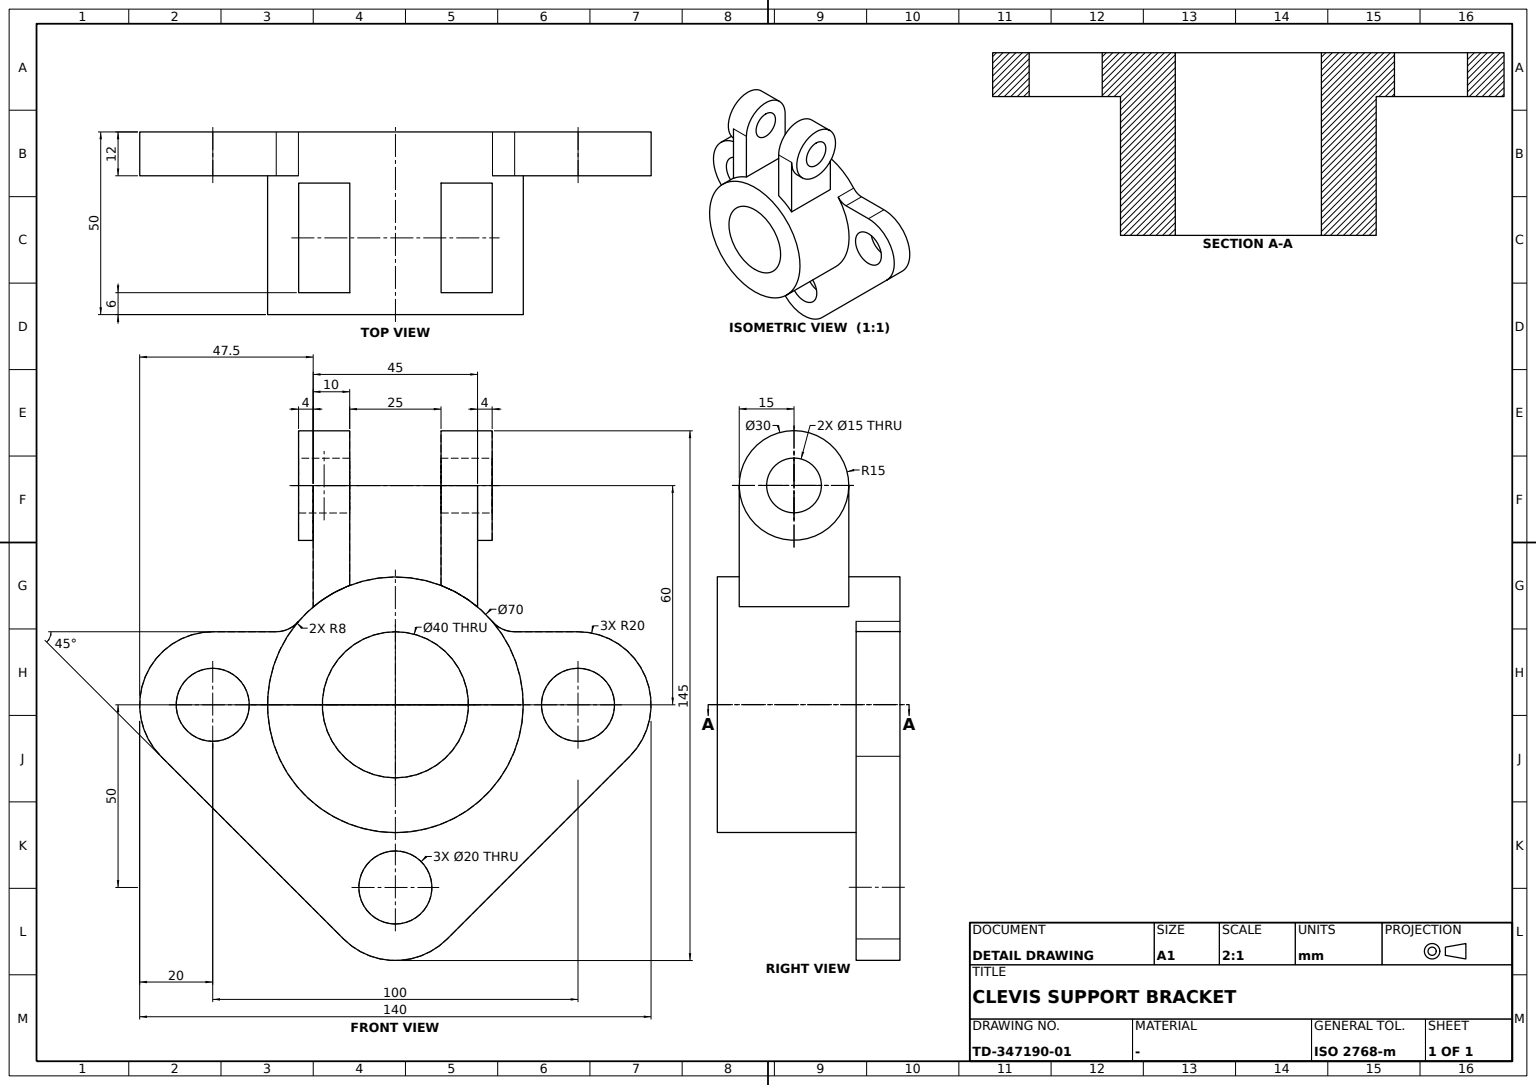
ISO-10303-21;
HEADER;
FILE_DESCRIPTION((''),'2;1');
FILE_NAME('','',(''),(''),'','','');
FILE_SCHEMA(('AUTOMOTIVE_DESIGN'));
ENDSEC;
DATA;
#1=APPLICATION_CONTEXT('');
#2=PRODUCT_CONTEXT('',#1,'mechanical');
#3=PRODUCT('','','',(#2));
#4=PRODUCT_DEFINITION_FORMATION('','',#3);
#5=PRODUCT_DEFINITION_CONTEXT('',#1,'design');
#6=PRODUCT_DEFINITION('','',#4,#5);
#7=PRODUCT_DEFINITION_SHAPE('','',#6);
#8=(LENGTH_UNIT()NAMED_UNIT(*)SI_UNIT(.MILLI.,.METRE.));
#9=(NAMED_UNIT(*)PLANE_ANGLE_UNIT()SI_UNIT($,.RADIAN.));
#10=(NAMED_UNIT(*)SI_UNIT($,.STERADIAN.)SOLID_ANGLE_UNIT());
#11=UNCERTAINTY_MEASURE_WITH_UNIT(LENGTH_MEASURE(0.005),#8,'distance_accuracy_value','');
#12=(GEOMETRIC_REPRESENTATION_CONTEXT(3)GLOBAL_UNCERTAINTY_ASSIGNED_CONTEXT((#11))GLOBAL_UNIT_ASSIGNED_CONTEXT((#8,#9,#10))REPRESENTATION_CONTEXT('',''));
#13=CARTESIAN_POINT('',(29.,-26.5,75.));
#14=VERTEX_POINT('',#13);
#15=CARTESIAN_POINT('',(29.,-26.5,60.));
#16=DIRECTION('',(0.,1.,0.));
#17=DIRECTION('',(0.,0.,1.));
#18=AXIS2_PLACEMENT_3D('',#15,#16,#17);
#19=CIRCLE('',#18,15.);
#20=EDGE_CURVE('',#14,#14,#19,.T.);
#21=ORIENTED_EDGE('',*,*,#20,.T.);
#22=EDGE_LOOP('',(#21));
#23=FACE_BOUND('',#22,.T.);
#24=CARTESIAN_POINT('',(44.,-22.5,60.));
#25=VERTEX_POINT('',#24);
#26=CARTESIAN_POINT('',(14.,-22.5,60.));
#27=VERTEX_POINT('',#26);
#28=CARTESIAN_POINT('',(29.,-22.5,60.));
#29=AXIS2_PLACEMENT_3D('',#28,#16,#17);
#30=CIRCLE('',#29,15.);
#31=EDGE_CURVE('',#25,#27,#30,.T.);
#32=ORIENTED_EDGE('',*,*,#31,.F.);
#33=CARTESIAN_POINT('',(44.,-12.5,60.));
#34=VERTEX_POINT('',#33);
#35=CARTESIAN_POINT('',(44.,24.5,60.));
#36=VECTOR('',#16,1000.);
#37=LINE('',#35,#36);
#38=EDGE_CURVE('',#25,#34,#37,.T.);
#39=ORIENTED_EDGE('',*,*,#38,.T.);
#40=CARTESIAN_POINT('',(14.,-12.5,60.));
#41=VERTEX_POINT('',#40);
#42=CARTESIAN_POINT('',(29.,-12.5,60.));
#43=DIRECTION('',(0.,-1.,0.));
#44=DIRECTION('',(0.,0.,-1.));
#45=AXIS2_PLACEMENT_3D('',#42,#43,#44);
#46=CIRCLE('',#45,15.);
#47=EDGE_CURVE('',#34,#41,#46,.T.);
#48=ORIENTED_EDGE('',*,*,#47,.T.);
#49=CARTESIAN_POINT('',(14.,24.5,60.));
#50=LINE('',#49,#36);
#51=EDGE_CURVE('',#27,#41,#50,.T.);
#52=ORIENTED_EDGE('',*,*,#51,.F.);
#53=EDGE_LOOP('',(#32,#39,#48,#52));
#54=FACE_BOUND('',#53,.T.);
#55=CARTESIAN_POINT('',(29.,24.5,60.));
#56=DIRECTION('',(-1.,0.,0.));
#57=AXIS2_PLACEMENT_3D('',#55,#16,#56);
#58=CYLINDRICAL_SURFACE('',#57,15.);
#59=ADVANCED_FACE('',(#23,#54),#58,.T.);
#60=CARTESIAN_POINT('',(29.,-12.5,52.5));
#61=VERTEX_POINT('',#60);
#62=CIRCLE('',#45,7.5);
#63=EDGE_CURVE('',#61,#61,#62,.T.);
#64=ORIENTED_EDGE('',*,*,#63,.F.);
#65=EDGE_LOOP('',(#64));
#66=FACE_BOUND('',#65,.T.);
#67=CARTESIAN_POINT('',(29.,-26.5,67.5));
#68=VERTEX_POINT('',#67);
#69=CIRCLE('',#18,7.5);
#70=EDGE_CURVE('',#68,#68,#69,.T.);
#71=ORIENTED_EDGE('',*,*,#70,.F.);
#72=EDGE_LOOP('',(#71));
#73=FACE_BOUND('',#72,.T.);
#74=CYLINDRICAL_SURFACE('',#57,7.5);
#75=ADVANCED_FACE('',(#66,#73),#74,.F.);
#76=CARTESIAN_POINT('',(29.,12.5,67.5));
#77=VERTEX_POINT('',#76);
#78=CARTESIAN_POINT('',(29.,12.5,60.));
#79=AXIS2_PLACEMENT_3D('',#78,#16,#17);
#80=CIRCLE('',#79,7.5);
#81=EDGE_CURVE('',#77,#77,#80,.T.);
#82=ORIENTED_EDGE('',*,*,#81,.T.);
#83=EDGE_LOOP('',(#82));
#84=FACE_BOUND('',#83,.T.);
#85=CARTESIAN_POINT('',(14.,12.5,60.));
#86=VERTEX_POINT('',#85);
#87=CARTESIAN_POINT('',(44.,12.5,60.));
#88=VERTEX_POINT('',#87);
#89=CIRCLE('',#79,15.);
#90=EDGE_CURVE('',#86,#88,#89,.T.);
#91=ORIENTED_EDGE('',*,*,#90,.F.);
#92=CARTESIAN_POINT('',(14.,12.5,32.691742));
#93=VERTEX_POINT('',#92);
#94=VECTOR('',#44,1000.);
#95=LINE('',#92,#94);
#96=EDGE_CURVE('',#86,#93,#95,.T.);
#97=ORIENTED_EDGE('',*,*,#96,.T.);
#98=CARTESIAN_POINT('',(44.,12.5,32.691742));
#99=VERTEX_POINT('',#98);
#100=DIRECTION('',(1.,0.,0.));
#101=VECTOR('',#100,1000.);
#102=LINE('',#92,#101);
#103=EDGE_CURVE('',#93,#99,#102,.T.);
#104=ORIENTED_EDGE('',*,*,#103,.T.);
#105=CARTESIAN_POINT('',(44.,12.5,25.));
#106=LINE('',#105,#94);
#107=EDGE_CURVE('',#88,#99,#106,.T.);
#108=ORIENTED_EDGE('',*,*,#107,.F.);
#109=EDGE_LOOP('',(#91,#97,#104,#108));
#110=FACE_BOUND('',#109,.T.);
#111=CARTESIAN_POINT('',(0.,12.5,32.691742));
#112=AXIS2_PLACEMENT_3D('',#111,#16,#17);
#113=PLANE('',#112);
#114=ADVANCED_FACE('',(#84,#110),#113,.F.);
#115=CARTESIAN_POINT('',(0.,-50.,20.));
#116=VERTEX_POINT('',#115);
#117=CARTESIAN_POINT('',(0.,-32.634338,20.));
#118=VERTEX_POINT('',#117);
#119=CARTESIAN_POINT('',(0.,0.,20.));
#120=LINE('',#119,#36);
#121=EDGE_CURVE('',#116,#118,#120,.T.);
#122=ORIENTED_EDGE('',*,*,#121,.F.);
#123=CARTESIAN_POINT('',(12.,-50.,20.));
#124=VERTEX_POINT('',#123);
#125=CARTESIAN_POINT('',(6.,-50.,20.));
#126=LINE('',#125,#101);
#127=EDGE_CURVE('',#116,#124,#126,.T.);
#128=ORIENTED_EDGE('',*,*,#127,.T.);
#129=CARTESIAN_POINT('',(12.,-32.634338,20.));
#130=VERTEX_POINT('',#129);
#131=CARTESIAN_POINT('',(12.,0.,20.));
#132=LINE('',#131,#36);
#133=EDGE_CURVE('',#124,#130,#132,.T.);
#134=ORIENTED_EDGE('',*,*,#133,.T.);
#135=CARTESIAN_POINT('',(6.,-32.634338,20.));
#136=LINE('',#135,#101);
#137=EDGE_CURVE('',#118,#130,#136,.T.);
#138=ORIENTED_EDGE('',*,*,#137,.F.);
#139=EDGE_LOOP('',(#122,#128,#134,#138));
#140=FACE_BOUND('',#139,.T.);
#141=CARTESIAN_POINT('',(0.,32.634338,20.));
#142=AXIS2_PLACEMENT_3D('',#141,#44,#16);
#143=PLANE('',#142);
#144=ADVANCED_FACE('',(#140),#143,.F.);
#145=CARTESIAN_POINT('',(44.,22.5,26.809513));
#146=VERTEX_POINT('',#145);
#147=CARTESIAN_POINT('',(44.,0.,0.));
#148=AXIS2_PLACEMENT_3D('',#147,#56,#17);
#149=CIRCLE('',#148,35.);
#150=EDGE_CURVE('',#99,#146,#149,.T.);
#151=ORIENTED_EDGE('',*,*,#150,.T.);
#152=CARTESIAN_POINT('',(44.,22.5,60.));
#153=VERTEX_POINT('',#152);
#154=CARTESIAN_POINT('',(44.,22.5,0.));
#155=VECTOR('',#17,1000.);
#156=LINE('',#154,#155);
#157=EDGE_CURVE('',#146,#153,#156,.T.);
#158=ORIENTED_EDGE('',*,*,#157,.T.);
#159=EDGE_CURVE('',#88,#153,#37,.T.);
#160=ORIENTED_EDGE('',*,*,#159,.F.);
#161=ORIENTED_EDGE('',*,*,#107,.T.);
#162=EDGE_LOOP('',(#151,#158,#160,#161));
#163=FACE_BOUND('',#162,.T.);
#164=CARTESIAN_POINT('',(44.,0.,25.));
#165=AXIS2_PLACEMENT_3D('',#164,#56,#17);
#166=PLANE('',#165);
#167=ADVANCED_FACE('',(#163),#166,.F.);
#168=ORIENTED_EDGE('',*,*,#31,.T.);
#169=CARTESIAN_POINT('',(14.,-22.5,26.809513));
#170=VERTEX_POINT('',#169);
#171=CARTESIAN_POINT('',(14.,-22.5,0.));
#172=LINE('',#171,#94);
#173=EDGE_CURVE('',#27,#170,#172,.T.);
#174=ORIENTED_EDGE('',*,*,#173,.T.);
#175=CARTESIAN_POINT('',(44.,-22.5,26.809513));
#176=VERTEX_POINT('',#175);
#177=LINE('',#175,#101);
#178=EDGE_CURVE('',#176,#170,#177,.F.);
#179=ORIENTED_EDGE('',*,*,#178,.F.);
#180=CARTESIAN_POINT('',(44.,-22.5,0.));
#181=LINE('',#180,#155);
#182=EDGE_CURVE('',#176,#25,#181,.T.);
#183=ORIENTED_EDGE('',*,*,#182,.T.);
#184=EDGE_LOOP('',(#168,#174,#179,#183));
#185=FACE_BOUND('',#184,.T.);
#186=CARTESIAN_POINT('',(0.,-22.5,0.));
#187=AXIS2_PLACEMENT_3D('',#186,#16,#56);
#188=PLANE('',#187);
#189=ADVANCED_FACE('',(#185),#188,.F.);
#190=CARTESIAN_POINT('',(0.,-50.,-10.));
#191=VERTEX_POINT('',#190);
#192=CARTESIAN_POINT('',(0.,-50.,0.));
#193=AXIS2_PLACEMENT_3D('',#192,#100,#44);
#194=CIRCLE('',#193,10.);
#195=EDGE_CURVE('',#191,#191,#194,.T.);
#196=ORIENTED_EDGE('',*,*,#195,.F.);
#197=EDGE_LOOP('',(#196));
#198=FACE_BOUND('',#197,.T.);
#199=CARTESIAN_POINT('',(12.,-50.,-10.));
#200=VERTEX_POINT('',#199);
#201=CARTESIAN_POINT('',(12.,-50.,0.));
#202=AXIS2_PLACEMENT_3D('',#201,#100,#44);
#203=CIRCLE('',#202,10.);
#204=EDGE_CURVE('',#200,#200,#203,.T.);
#205=ORIENTED_EDGE('',*,*,#204,.T.);
#206=EDGE_LOOP('',(#205));
#207=FACE_BOUND('',#206,.T.);
#208=CARTESIAN_POINT('',(6.,-50.,0.));
#209=AXIS2_PLACEMENT_3D('',#208,#100,#16);
#210=CYLINDRICAL_SURFACE('',#209,10.);
#211=ADVANCED_FACE('',(#198,#207),#210,.F.);
#212=CARTESIAN_POINT('',(0.,-14.142136,-64.142136));
#213=VERTEX_POINT('',#212);
#214=CARTESIAN_POINT('',(0.,14.142136,-64.142136));
#215=VERTEX_POINT('',#214);
#216=CARTESIAN_POINT('',(0.,0.,-50.));
#217=AXIS2_PLACEMENT_3D('',#216,#100,#44);
#218=CIRCLE('',#217,20.);
#219=EDGE_CURVE('',#213,#215,#218,.T.);
#220=ORIENTED_EDGE('',*,*,#219,.T.);
#221=CARTESIAN_POINT('',(12.,14.142136,-64.142136));
#222=VERTEX_POINT('',#221);
#223=CARTESIAN_POINT('',(6.,14.142136,-64.142136));
#224=LINE('',#223,#101);
#225=EDGE_CURVE('',#215,#222,#224,.T.);
#226=ORIENTED_EDGE('',*,*,#225,.T.);
#227=CARTESIAN_POINT('',(12.,-14.142136,-64.142136));
#228=VERTEX_POINT('',#227);
#229=CARTESIAN_POINT('',(12.,0.,-50.));
#230=AXIS2_PLACEMENT_3D('',#229,#100,#44);
#231=CIRCLE('',#230,20.);
#232=EDGE_CURVE('',#228,#222,#231,.T.);
#233=ORIENTED_EDGE('',*,*,#232,.F.);
#234=CARTESIAN_POINT('',(6.,-14.142136,-64.142136));
#235=LINE('',#234,#101);
#236=EDGE_CURVE('',#213,#228,#235,.T.);
#237=ORIENTED_EDGE('',*,*,#236,.F.);
#238=EDGE_LOOP('',(#220,#226,#233,#237));
#239=FACE_BOUND('',#238,.T.);
#240=CARTESIAN_POINT('',(6.,0.,-50.));
#241=AXIS2_PLACEMENT_3D('',#240,#100,#16);
#242=CYLINDRICAL_SURFACE('',#241,20.);
#243=ADVANCED_FACE('',(#239),#242,.T.);
#244=CARTESIAN_POINT('',(0.,-26.562833,22.790698));
#245=VERTEX_POINT('',#244);
#246=CARTESIAN_POINT('',(12.,-26.562833,22.790698));
#247=VERTEX_POINT('',#246);
#248=CARTESIAN_POINT('',(6.,-26.562833,22.790698));
#249=LINE('',#248,#101);
#250=EDGE_CURVE('',#245,#247,#249,.T.);
#251=ORIENTED_EDGE('',*,*,#250,.T.);
#252=CARTESIAN_POINT('',(12.,26.562833,22.790698));
#253=VERTEX_POINT('',#252);
#254=CARTESIAN_POINT('',(12.,0.,0.));
#255=AXIS2_PLACEMENT_3D('',#254,#100,#44);
#256=CIRCLE('',#255,35.);
#257=EDGE_CURVE('',#247,#253,#256,.T.);
#258=ORIENTED_EDGE('',*,*,#257,.T.);
#259=CARTESIAN_POINT('',(0.,26.562833,22.790698));
#260=VERTEX_POINT('',#259);
#261=CARTESIAN_POINT('',(6.,26.562833,22.790698));
#262=LINE('',#261,#101);
#263=EDGE_CURVE('',#260,#253,#262,.T.);
#264=ORIENTED_EDGE('',*,*,#263,.F.);
#265=CARTESIAN_POINT('',(0.,0.,0.));
#266=AXIS2_PLACEMENT_3D('',#265,#100,#44);
#267=CIRCLE('',#266,35.);
#268=EDGE_CURVE('',#260,#245,#267,.T.);
#269=ORIENTED_EDGE('',*,*,#268,.T.);
#270=EDGE_LOOP('',(#251,#258,#264,#269));
#271=FACE_BOUND('',#270,.T.);
#272=CARTESIAN_POINT('',(50.,0.,-35.));
#273=VERTEX_POINT('',#272);
#274=CARTESIAN_POINT('',(50.,0.,0.));
#275=AXIS2_PLACEMENT_3D('',#274,#100,#44);
#276=CIRCLE('',#275,35.);
#277=EDGE_CURVE('',#273,#273,#276,.T.);
#278=ORIENTED_EDGE('',*,*,#277,.F.);
#279=EDGE_LOOP('',(#278));
#280=FACE_BOUND('',#279,.T.);
#281=CARTESIAN_POINT('',(14.,22.5,26.809513));
#282=VERTEX_POINT('',#281);
#283=LINE('',#145,#101);
#284=EDGE_CURVE('',#146,#282,#283,.F.);
#285=ORIENTED_EDGE('',*,*,#284,.F.);
#286=ORIENTED_EDGE('',*,*,#150,.F.);
#287=ORIENTED_EDGE('',*,*,#103,.F.);
#288=CARTESIAN_POINT('',(14.,0.,0.));
#289=AXIS2_PLACEMENT_3D('',#288,#100,#44);
#290=CIRCLE('',#289,35.);
#291=EDGE_CURVE('',#282,#93,#290,.T.);
#292=ORIENTED_EDGE('',*,*,#291,.F.);
#293=EDGE_LOOP('',(#285,#286,#287,#292));
#294=FACE_BOUND('',#293,.T.);
#295=CARTESIAN_POINT('',(14.,-12.5,32.691742));
#296=VERTEX_POINT('',#295);
#297=EDGE_CURVE('',#296,#170,#290,.T.);
#298=ORIENTED_EDGE('',*,*,#297,.F.);
#299=CARTESIAN_POINT('',(44.,-12.5,32.691742));
#300=VERTEX_POINT('',#299);
#301=LINE('',#295,#101);
#302=EDGE_CURVE('',#296,#300,#301,.T.);
#303=ORIENTED_EDGE('',*,*,#302,.T.);
#304=EDGE_CURVE('',#176,#300,#149,.T.);
#305=ORIENTED_EDGE('',*,*,#304,.F.);
#306=ORIENTED_EDGE('',*,*,#178,.T.);
#307=EDGE_LOOP('',(#298,#303,#305,#306));
#308=FACE_BOUND('',#307,.T.);
#309=CARTESIAN_POINT('',(25.,0.,0.));
#310=AXIS2_PLACEMENT_3D('',#309,#100,#16);
#311=CYLINDRICAL_SURFACE('',#310,35.);
#312=ADVANCED_FACE('',(#271,#280,#294,#308),#311,.T.);
#313=ORIENTED_EDGE('',*,*,#20,.F.);
#314=EDGE_LOOP('',(#313));
#315=FACE_BOUND('',#314,.T.);
#316=ORIENTED_EDGE('',*,*,#70,.T.);
#317=EDGE_LOOP('',(#316));
#318=FACE_BOUND('',#317,.T.);
#319=CARTESIAN_POINT('',(0.,-26.5,0.));
#320=AXIS2_PLACEMENT_3D('',#319,#16,#56);
#321=PLANE('',#320);
#322=ADVANCED_FACE('',(#315,#318),#321,.F.);
#323=CARTESIAN_POINT('',(0.,0.,-60.));
#324=VERTEX_POINT('',#323);
#325=CIRCLE('',#217,10.);
#326=EDGE_CURVE('',#324,#324,#325,.T.);
#327=ORIENTED_EDGE('',*,*,#326,.F.);
#328=EDGE_LOOP('',(#327));
#329=FACE_BOUND('',#328,.T.);
#330=CARTESIAN_POINT('',(12.,0.,-60.));
#331=VERTEX_POINT('',#330);
#332=CIRCLE('',#230,10.);
#333=EDGE_CURVE('',#331,#331,#332,.T.);
#334=ORIENTED_EDGE('',*,*,#333,.T.);
#335=EDGE_LOOP('',(#334));
#336=FACE_BOUND('',#335,.T.);
#337=CYLINDRICAL_SURFACE('',#241,10.);
#338=ADVANCED_FACE('',(#329,#336),#337,.F.);
#339=CARTESIAN_POINT('',(0.,50.,20.));
#340=VERTEX_POINT('',#339);
#341=CARTESIAN_POINT('',(12.,50.,20.));
#342=VERTEX_POINT('',#341);
#343=CARTESIAN_POINT('',(6.,50.,20.));
#344=LINE('',#343,#101);
#345=EDGE_CURVE('',#340,#342,#344,.T.);
#346=ORIENTED_EDGE('',*,*,#345,.F.);
#347=VERTEX_POINT('',#141);
#348=EDGE_CURVE('',#347,#340,#120,.T.);
#349=ORIENTED_EDGE('',*,*,#348,.F.);
#350=CARTESIAN_POINT('',(12.,32.634338,20.));
#351=VERTEX_POINT('',#350);
#352=CARTESIAN_POINT('',(6.,32.634338,20.));
#353=LINE('',#352,#101);
#354=EDGE_CURVE('',#347,#351,#353,.T.);
#355=ORIENTED_EDGE('',*,*,#354,.T.);
#356=EDGE_CURVE('',#351,#342,#132,.T.);
#357=ORIENTED_EDGE('',*,*,#356,.T.);
#358=EDGE_LOOP('',(#346,#349,#355,#357));
#359=FACE_BOUND('',#358,.T.);
#360=ADVANCED_FACE('',(#359),#143,.F.);
#361=ORIENTED_EDGE('',*,*,#159,.T.);
#362=CARTESIAN_POINT('',(14.,22.5,60.));
#363=VERTEX_POINT('',#362);
#364=CARTESIAN_POINT('',(29.,22.5,60.));
#365=AXIS2_PLACEMENT_3D('',#364,#16,#17);
#366=CIRCLE('',#365,15.);
#367=EDGE_CURVE('',#153,#363,#366,.T.);
#368=ORIENTED_EDGE('',*,*,#367,.T.);
#369=EDGE_CURVE('',#86,#363,#50,.T.);
#370=ORIENTED_EDGE('',*,*,#369,.F.);
#371=ORIENTED_EDGE('',*,*,#90,.T.);
#372=EDGE_LOOP('',(#361,#368,#370,#371));
#373=FACE_BOUND('',#372,.T.);
#374=CARTESIAN_POINT('',(29.,26.5,75.));
#375=VERTEX_POINT('',#374);
#376=CARTESIAN_POINT('',(29.,26.5,60.));
#377=AXIS2_PLACEMENT_3D('',#376,#16,#17);
#378=CIRCLE('',#377,15.);
#379=EDGE_CURVE('',#375,#375,#378,.T.);
#380=ORIENTED_EDGE('',*,*,#379,.F.);
#381=EDGE_LOOP('',(#380));
#382=FACE_BOUND('',#381,.T.);
#383=ADVANCED_FACE('',(#373,#382),#58,.T.);
#384=CARTESIAN_POINT('',(0.,0.,-20.));
#385=VERTEX_POINT('',#384);
#386=CIRCLE('',#266,20.);
#387=EDGE_CURVE('',#385,#385,#386,.T.);
#388=ORIENTED_EDGE('',*,*,#387,.T.);
#389=EDGE_LOOP('',(#388));
#390=FACE_BOUND('',#389,.T.);
#391=ORIENTED_EDGE('',*,*,#326,.T.);
#392=EDGE_LOOP('',(#391));
#393=FACE_BOUND('',#392,.T.);
#394=ORIENTED_EDGE('',*,*,#195,.T.);
#395=EDGE_LOOP('',(#394));
#396=FACE_BOUND('',#395,.T.);
#397=ORIENTED_EDGE('',*,*,#268,.F.);
#398=CARTESIAN_POINT('',(0.,32.634338,28.));
#399=AXIS2_PLACEMENT_3D('',#398,#100,#44);
#400=CIRCLE('',#399,8.);
#401=EDGE_CURVE('',#260,#347,#400,.T.);
#402=ORIENTED_EDGE('',*,*,#401,.T.);
#403=ORIENTED_EDGE('',*,*,#348,.T.);
#404=CARTESIAN_POINT('',(0.,64.142136,-14.142136));
#405=VERTEX_POINT('',#404);
#406=CARTESIAN_POINT('',(0.,50.,0.));
#407=AXIS2_PLACEMENT_3D('',#406,#100,#44);
#408=CIRCLE('',#407,20.);
#409=EDGE_CURVE('',#405,#340,#408,.T.);
#410=ORIENTED_EDGE('',*,*,#409,.F.);
#411=CARTESIAN_POINT('',(0.,39.142136,-39.142136));
#412=DIRECTION('',(0.,0.707106781,0.707106781));
#413=VECTOR('',#412,1000.);
#414=LINE('',#411,#413);
#415=EDGE_CURVE('',#215,#405,#414,.T.);
#416=ORIENTED_EDGE('',*,*,#415,.F.);
#417=ORIENTED_EDGE('',*,*,#219,.F.);
#418=CARTESIAN_POINT('',(0.,-64.142136,-14.142136));
#419=VERTEX_POINT('',#418);
#420=CARTESIAN_POINT('',(0.,-39.142136,-39.142136));
#421=DIRECTION('',(0.,0.707106781,-0.707106781));
#422=VECTOR('',#421,1000.);
#423=LINE('',#420,#422);
#424=EDGE_CURVE('',#419,#213,#423,.T.);
#425=ORIENTED_EDGE('',*,*,#424,.F.);
#426=CIRCLE('',#193,20.);
#427=EDGE_CURVE('',#116,#419,#426,.T.);
#428=ORIENTED_EDGE('',*,*,#427,.F.);
#429=ORIENTED_EDGE('',*,*,#121,.T.);
#430=CARTESIAN_POINT('',(0.,-32.634338,28.));
#431=AXIS2_PLACEMENT_3D('',#430,#100,#44);
#432=CIRCLE('',#431,8.);
#433=EDGE_CURVE('',#118,#245,#432,.T.);
#434=ORIENTED_EDGE('',*,*,#433,.T.);
#435=EDGE_LOOP('',(#397,#402,#403,#410,#416,#417,#425,#428,#429,#434));
#436=FACE_BOUND('',#435,.T.);
#437=CARTESIAN_POINT('',(0.,50.,-10.));
#438=VERTEX_POINT('',#437);
#439=CIRCLE('',#407,10.);
#440=EDGE_CURVE('',#438,#438,#439,.T.);
#441=ORIENTED_EDGE('',*,*,#440,.T.);
#442=EDGE_LOOP('',(#441));
#443=FACE_BOUND('',#442,.T.);
#444=AXIS2_PLACEMENT_3D('',#265,#100,#16);
#445=PLANE('',#444);
#446=ADVANCED_FACE('',(#390,#393,#396,#436,#443),#445,.F.);
#447=CARTESIAN_POINT('',(44.,-12.5,91.649002));
#448=LINE('',#447,#94);
#449=EDGE_CURVE('',#34,#300,#448,.T.);
#450=ORIENTED_EDGE('',*,*,#449,.F.);
#451=ORIENTED_EDGE('',*,*,#38,.F.);
#452=ORIENTED_EDGE('',*,*,#182,.F.);
#453=ORIENTED_EDGE('',*,*,#304,.T.);
#454=EDGE_LOOP('',(#450,#451,#452,#453));
#455=FACE_BOUND('',#454,.T.);
#456=ADVANCED_FACE('',(#455),#166,.F.);
#457=CARTESIAN_POINT('',(50.,0.,-20.));
#458=VERTEX_POINT('',#457);
#459=CIRCLE('',#275,20.);
#460=EDGE_CURVE('',#458,#458,#459,.T.);
#461=ORIENTED_EDGE('',*,*,#460,.F.);
#462=EDGE_LOOP('',(#461));
#463=FACE_BOUND('',#462,.T.);
#464=ORIENTED_EDGE('',*,*,#277,.T.);
#465=EDGE_LOOP('',(#464));
#466=FACE_BOUND('',#465,.T.);
#467=AXIS2_PLACEMENT_3D('',#274,#100,#16);
#468=PLANE('',#467);
#469=ADVANCED_FACE('',(#463,#466),#468,.T.);
#470=CARTESIAN_POINT('',(12.,50.,-10.));
#471=VERTEX_POINT('',#470);
#472=CARTESIAN_POINT('',(12.,50.,0.));
#473=AXIS2_PLACEMENT_3D('',#472,#100,#44);
#474=CIRCLE('',#473,10.);
#475=EDGE_CURVE('',#471,#471,#474,.T.);
#476=ORIENTED_EDGE('',*,*,#475,.T.);
#477=EDGE_LOOP('',(#476));
#478=FACE_BOUND('',#477,.T.);
#479=ORIENTED_EDGE('',*,*,#440,.F.);
#480=EDGE_LOOP('',(#479));
#481=FACE_BOUND('',#480,.T.);
#482=CARTESIAN_POINT('',(6.,50.,0.));
#483=AXIS2_PLACEMENT_3D('',#482,#100,#16);
#484=CYLINDRICAL_SURFACE('',#483,10.);
#485=ADVANCED_FACE('',(#478,#481),#484,.F.);
#486=ORIENTED_EDGE('',*,*,#291,.T.);
#487=ORIENTED_EDGE('',*,*,#96,.F.);
#488=ORIENTED_EDGE('',*,*,#369,.T.);
#489=CARTESIAN_POINT('',(14.,22.5,0.));
#490=LINE('',#489,#94);
#491=EDGE_CURVE('',#363,#282,#490,.T.);
#492=ORIENTED_EDGE('',*,*,#491,.T.);
#493=EDGE_LOOP('',(#486,#487,#488,#492));
#494=FACE_BOUND('',#493,.T.);
#495=CARTESIAN_POINT('',(14.,0.,60.));
#496=AXIS2_PLACEMENT_3D('',#495,#100,#44);
#497=PLANE('',#496);
#498=ADVANCED_FACE('',(#494),#497,.F.);
#499=LINE('',#40,#94);
#500=EDGE_CURVE('',#41,#296,#499,.T.);
#501=ORIENTED_EDGE('',*,*,#500,.T.);
#502=ORIENTED_EDGE('',*,*,#297,.T.);
#503=ORIENTED_EDGE('',*,*,#173,.F.);
#504=ORIENTED_EDGE('',*,*,#51,.T.);
#505=EDGE_LOOP('',(#501,#502,#503,#504));
#506=FACE_BOUND('',#505,.T.);
#507=ADVANCED_FACE('',(#506),#497,.F.);
#508=CARTESIAN_POINT('',(12.,64.142136,-14.142136));
#509=VERTEX_POINT('',#508);
#510=CARTESIAN_POINT('',(12.,39.142136,-39.142136));
#511=LINE('',#510,#413);
#512=EDGE_CURVE('',#222,#509,#511,.T.);
#513=ORIENTED_EDGE('',*,*,#512,.F.);
#514=ORIENTED_EDGE('',*,*,#225,.F.);
#515=ORIENTED_EDGE('',*,*,#415,.T.);
#516=CARTESIAN_POINT('',(6.,64.142136,-14.142136));
#517=LINE('',#516,#101);
#518=EDGE_CURVE('',#405,#509,#517,.T.);
#519=ORIENTED_EDGE('',*,*,#518,.T.);
#520=EDGE_LOOP('',(#513,#514,#515,#519));
#521=FACE_BOUND('',#520,.T.);
#522=AXIS2_PLACEMENT_3D('',#214,#421,#412);
#523=PLANE('',#522);
#524=ADVANCED_FACE('',(#521),#523,.T.);
#525=CARTESIAN_POINT('',(29.,26.5,67.5));
#526=VERTEX_POINT('',#525);
#527=CIRCLE('',#377,7.5);
#528=EDGE_CURVE('',#526,#526,#527,.T.);
#529=ORIENTED_EDGE('',*,*,#528,.T.);
#530=EDGE_LOOP('',(#529));
#531=FACE_BOUND('',#530,.T.);
#532=ORIENTED_EDGE('',*,*,#81,.F.);
#533=EDGE_LOOP('',(#532));
#534=FACE_BOUND('',#533,.T.);
#535=ADVANCED_FACE('',(#531,#534),#74,.F.);
#536=ORIENTED_EDGE('',*,*,#250,.F.);
#537=ORIENTED_EDGE('',*,*,#433,.F.);
#538=ORIENTED_EDGE('',*,*,#137,.T.);
#539=CARTESIAN_POINT('',(12.,-32.634338,28.));
#540=AXIS2_PLACEMENT_3D('',#539,#100,#44);
#541=CIRCLE('',#540,8.);
#542=EDGE_CURVE('',#130,#247,#541,.T.);
#543=ORIENTED_EDGE('',*,*,#542,.T.);
#544=EDGE_LOOP('',(#536,#537,#538,#543));
#545=FACE_BOUND('',#544,.T.);
#546=CARTESIAN_POINT('',(6.,-32.634338,28.));
#547=AXIS2_PLACEMENT_3D('',#546,#100,#16);
#548=CYLINDRICAL_SURFACE('',#547,8.);
#549=ADVANCED_FACE('',(#545),#548,.F.);
#550=ORIENTED_EDGE('',*,*,#518,.F.);
#551=ORIENTED_EDGE('',*,*,#409,.T.);
#552=ORIENTED_EDGE('',*,*,#345,.T.);
#553=CIRCLE('',#473,20.);
#554=EDGE_CURVE('',#509,#342,#553,.T.);
#555=ORIENTED_EDGE('',*,*,#554,.F.);
#556=EDGE_LOOP('',(#550,#551,#552,#555));
#557=FACE_BOUND('',#556,.T.);
#558=CYLINDRICAL_SURFACE('',#483,20.);
#559=ADVANCED_FACE('',(#557),#558,.T.);
#560=ORIENTED_EDGE('',*,*,#449,.T.);
#561=ORIENTED_EDGE('',*,*,#302,.F.);
#562=ORIENTED_EDGE('',*,*,#500,.F.);
#563=ORIENTED_EDGE('',*,*,#47,.F.);
#564=EDGE_LOOP('',(#560,#561,#562,#563));
#565=FACE_BOUND('',#564,.T.);
#566=ORIENTED_EDGE('',*,*,#63,.T.);
#567=EDGE_LOOP('',(#566));
#568=FACE_BOUND('',#567,.T.);
#569=CARTESIAN_POINT('',(0.,-12.5,91.649002));
#570=AXIS2_PLACEMENT_3D('',#569,#43,#44);
#571=PLANE('',#570);
#572=ADVANCED_FACE('',(#565,#568),#571,.F.);
#573=ORIENTED_EDGE('',*,*,#157,.F.);
#574=ORIENTED_EDGE('',*,*,#284,.T.);
#575=ORIENTED_EDGE('',*,*,#491,.F.);
#576=ORIENTED_EDGE('',*,*,#367,.F.);
#577=EDGE_LOOP('',(#573,#574,#575,#576));
#578=FACE_BOUND('',#577,.T.);
#579=CARTESIAN_POINT('',(0.,22.5,0.));
#580=AXIS2_PLACEMENT_3D('',#579,#16,#56);
#581=PLANE('',#580);
#582=ADVANCED_FACE('',(#578),#581,.T.);
#583=ORIENTED_EDGE('',*,*,#460,.T.);
#584=EDGE_LOOP('',(#583));
#585=FACE_BOUND('',#584,.T.);
#586=ORIENTED_EDGE('',*,*,#387,.F.);
#587=EDGE_LOOP('',(#586));
#588=FACE_BOUND('',#587,.T.);
#589=CARTESIAN_POINT('',(6.,0.,0.));
#590=AXIS2_PLACEMENT_3D('',#589,#100,#16);
#591=CYLINDRICAL_SURFACE('',#590,20.);
#592=ADVANCED_FACE('',(#585,#588),#591,.F.);
#593=ORIENTED_EDGE('',*,*,#263,.T.);
#594=CARTESIAN_POINT('',(12.,32.634338,28.));
#595=AXIS2_PLACEMENT_3D('',#594,#100,#44);
#596=CIRCLE('',#595,8.);
#597=EDGE_CURVE('',#253,#351,#596,.T.);
#598=ORIENTED_EDGE('',*,*,#597,.T.);
#599=ORIENTED_EDGE('',*,*,#354,.F.);
#600=ORIENTED_EDGE('',*,*,#401,.F.);
#601=EDGE_LOOP('',(#593,#598,#599,#600));
#602=FACE_BOUND('',#601,.T.);
#603=CARTESIAN_POINT('',(6.,32.634338,28.));
#604=AXIS2_PLACEMENT_3D('',#603,#100,#16);
#605=CYLINDRICAL_SURFACE('',#604,8.);
#606=ADVANCED_FACE('',(#602),#605,.F.);
#607=ORIENTED_EDGE('',*,*,#379,.T.);
#608=EDGE_LOOP('',(#607));
#609=FACE_BOUND('',#608,.T.);
#610=ORIENTED_EDGE('',*,*,#528,.F.);
#611=EDGE_LOOP('',(#610));
#612=FACE_BOUND('',#611,.T.);
#613=CARTESIAN_POINT('',(0.,26.5,0.));
#614=AXIS2_PLACEMENT_3D('',#613,#16,#56);
#615=PLANE('',#614);
#616=ADVANCED_FACE('',(#609,#612),#615,.T.);
#617=CARTESIAN_POINT('',(12.,-64.142136,-14.142136));
#618=VERTEX_POINT('',#617);
#619=CARTESIAN_POINT('',(6.,-64.142136,-14.142136));
#620=LINE('',#619,#101);
#621=EDGE_CURVE('',#419,#618,#620,.T.);
#622=ORIENTED_EDGE('',*,*,#621,.T.);
#623=CIRCLE('',#202,20.);
#624=EDGE_CURVE('',#124,#618,#623,.T.);
#625=ORIENTED_EDGE('',*,*,#624,.F.);
#626=ORIENTED_EDGE('',*,*,#127,.F.);
#627=ORIENTED_EDGE('',*,*,#427,.T.);
#628=EDGE_LOOP('',(#622,#625,#626,#627));
#629=FACE_BOUND('',#628,.T.);
#630=CYLINDRICAL_SURFACE('',#209,20.);
#631=ADVANCED_FACE('',(#629),#630,.T.);
#632=ORIENTED_EDGE('',*,*,#424,.T.);
#633=ORIENTED_EDGE('',*,*,#236,.T.);
#634=CARTESIAN_POINT('',(12.,-39.142136,-39.142136));
#635=LINE('',#634,#422);
#636=EDGE_CURVE('',#618,#228,#635,.T.);
#637=ORIENTED_EDGE('',*,*,#636,.F.);
#638=ORIENTED_EDGE('',*,*,#621,.F.);
#639=EDGE_LOOP('',(#632,#633,#637,#638));
#640=FACE_BOUND('',#639,.T.);
#641=DIRECTION('',(0.,-0.707106781,-0.707106781));
#642=AXIS2_PLACEMENT_3D('',#418,#641,#421);
#643=PLANE('',#642);
#644=ADVANCED_FACE('',(#640),#643,.T.);
#645=ORIENTED_EDGE('',*,*,#597,.F.);
#646=ORIENTED_EDGE('',*,*,#257,.F.);
#647=ORIENTED_EDGE('',*,*,#542,.F.);
#648=ORIENTED_EDGE('',*,*,#133,.F.);
#649=ORIENTED_EDGE('',*,*,#624,.T.);
#650=ORIENTED_EDGE('',*,*,#636,.T.);
#651=ORIENTED_EDGE('',*,*,#232,.T.);
#652=ORIENTED_EDGE('',*,*,#512,.T.);
#653=ORIENTED_EDGE('',*,*,#554,.T.);
#654=ORIENTED_EDGE('',*,*,#356,.F.);
#655=EDGE_LOOP('',(#645,#646,#647,#648,#649,#650,#651,#652,#653,#654));
#656=FACE_BOUND('',#655,.T.);
#657=ORIENTED_EDGE('',*,*,#204,.F.);
#658=EDGE_LOOP('',(#657));
#659=FACE_BOUND('',#658,.T.);
#660=ORIENTED_EDGE('',*,*,#333,.F.);
#661=EDGE_LOOP('',(#660));
#662=FACE_BOUND('',#661,.T.);
#663=ORIENTED_EDGE('',*,*,#475,.F.);
#664=EDGE_LOOP('',(#663));
#665=FACE_BOUND('',#664,.T.);
#666=AXIS2_PLACEMENT_3D('',#254,#100,#16);
#667=PLANE('',#666);
#668=ADVANCED_FACE('',(#656,#659,#662,#665),#667,.T.);
#669=CLOSED_SHELL('',(#59,#75,#114,#144,#167,#189,#211,#243,#312,#322,#338,#360,#383,#446,#456,#469,#485,#498,#507,#524,#535,#549,#559,#572,#582,#592,#606,#616,#631,#644,#668));
#670=MANIFOLD_SOLID_BREP('',#669);
#671=ADVANCED_BREP_SHAPE_REPRESENTATION('',(#670),#12);
#672=SHAPE_DEFINITION_REPRESENTATION(#7,#671);
ENDSEC;
END-ISO-10303-21;
